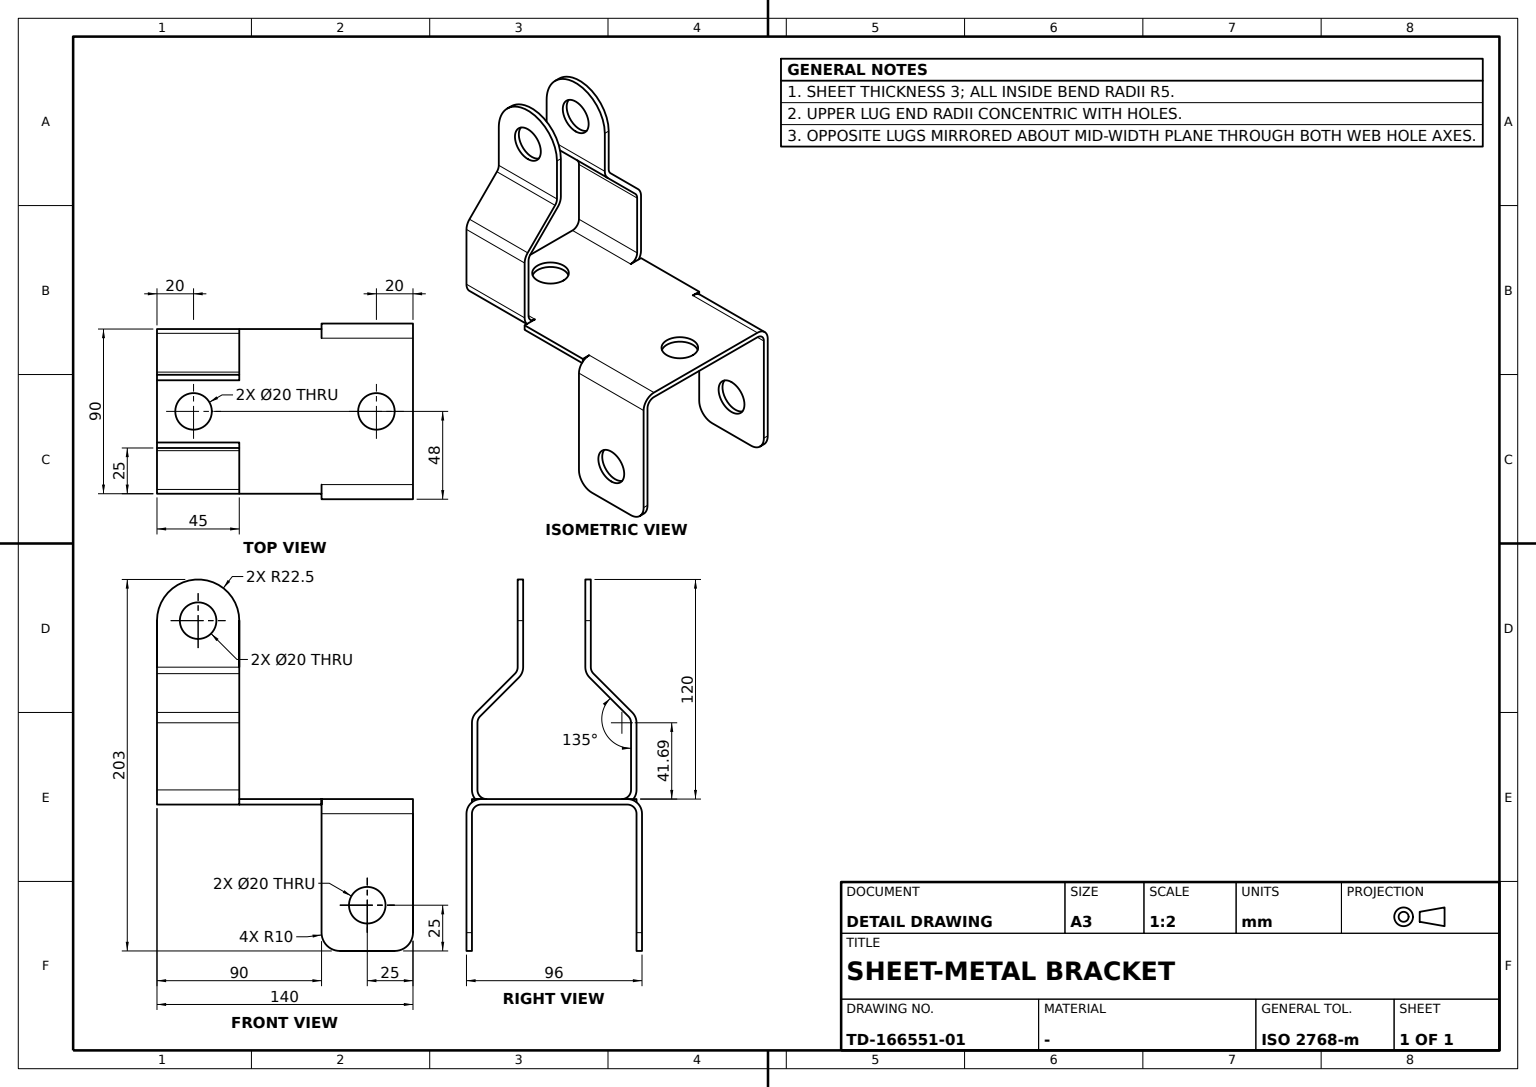
solid
v1 (60,0,1.5)
e1 v1 v1 CIRCLE(AX(P(50,0,1.5),D(0,0,1),D(1,0,0)),10)
v2 (60,0,-1.5)
e2 v2 v2 CIRCLE(AX(P(50,0,-1.5),D(0,0,1),D(1,0,0)),10)
face CYL(AX(P(50,0,-1.5),D(0,0,1),D(1,0,0)),10) rev [e1] [-e2]
v3 (45,48,-46.5)
e3 v3 v3 CIRCLE(AX(P(45,48,-56.5),D(0,1,0),D(0,0,1)),10) rev
v4 (45,45,-46.5)
e4 v4 v4 CIRCLE(AX(P(45,45,-56.5),D(0,1,0),D(0,0,1)),10)
face CYL(AX(P(45,48,-56.5),D(0,1,0),D(1,0,0)),10) rev [-e3] [-e4]
v5 (-25,-45,43.186292)
v6 (-70,-45,43.186292)
e5 v5 v6 LINE
v7 (-70,-45,6.5)
e6 v7 v6 LINE
v8 (-25,-45,6.5)
e7 v8 v7 LINE
e8 v8 v5 LINE
face PLANE(AX(P(-70,-45,1.5),D(0,-1,0),D(0,0,1))) [e5 -e6 -e7 e8]
v9 (30.000004,-45,-81.5)
v10 (60,-45,-81.5)
e9 v9 v10 LINE
v11 (60,-48,-81.5)
e10 v10 v11 LINE
v12 (30,-48,-81.5)
e11 v11 v12 LINE
e12 v9 v12 LINE
face PLANE(AX(P(45,48,-81.5),D(0,0,1),D(1,0,0))) rev [e9 e10 e11 -e12]
v13 (-70,-20,73.571068)
v14 (-70,-20,99)
e13 v13 v14 LINE
v15 (-25,-20,73.571068)
e14 v15 v13 LINE
v16 (-25,-20,99)
e15 v15 v16 LINE
e16 v16 v14 CIRCLE(AX(P(-47.5,-20,99),D(0,-1,0),D(0,0,-1)),22.5)
v17 (-47.5,-20,89)
e17 v17 v17 CIRCLE(AX(P(-47.5,-20,99),D(0,-1,0),D(0,0,-1)),10)
face PLANE(AX(P(-70,-20,71.5),D(0,-1,0),D(0,0,1))) [-e13 -e14 e15 e16] [-e17]
v18 (30,48,-81.5)
v19 (60,48,-81.5)
e18 v18 v19 LINE
v20 (20,48,-71.5)
e19 v18 v20 CIRCLE(AX(P(30,48,-71.5),D(0,1,0),D(0,0,1)),10)
v21 (20,48,-6.5)
e20 v20 v21 LINE
v22 (70,48,-6.5)
e21 v21 v22 LINE
v23 (70,48,-71.5)
e22 v23 v22 LINE
e23 v23 v19 CIRCLE(AX(P(60,48,-71.5),D(0,1,0),D(0,0,1)),10)
face PLANE(AX(P(0,48,-1.5),D(0,1,0),D(1,0,0))) [e3] [-e18 e19 e20 e21 -e22 e23]
v24 (20,-40,-1.5)
v25 (20,-45,-6.5)
e24 v24 v25 CIRCLE(AX(P(20,-40,-6.5),D(1,0,0),D(0,1,0)),5)
v26 (70,-40,-1.5)
e25 v26 v24 LINE
v27 (70,-45,-6.5)
e26 v27 v26 CIRCLE(AX(P(70,-40,-6.5),D(-1,0,0),D(0,0,1)),5)
e27 v27 v25 LINE
face CYL(AX(P(0,-40,-6.5),D(-1,0,0),D(0,0,1)),5) rev [-e24 -e25 -e26 e27]
v28 (-25,-42.656854,48.843146)
e28 v28 v5 CIRCLE(AX(P(-25,-37,43.186292),D(-1,0,0),D(0,0,1)),8) rev
v29 (-70,-42.656854,48.843146)
e29 v28 v29 LINE
e30 v6 v29 CIRCLE(AX(P(-70,-37,43.186292),D(-1,0,0),D(0,0,1)),8)
face CYL(AX(P(-47.5,-37,43.186292),D(1,0,0),D(0,-1,0)),8) [-e5 -e28 e29 -e30]
v30 (-70,-17,99)
e31 v14 v30 LINE
v31 (-25,-17,99)
e32 v16 v31 LINE
e33 v31 v30 CIRCLE(AX(P(-47.5,-17,99),D(0,-1,0),D(0,0,-1)),22.5)
face CYL(AX(P(-47.5,-20,99),D(0,-1,0),D(0,0,1)),22.5) [-e31 -e16 e32 e33]
v32 (-25,-37,-1.5)
v33 (-25,-37,1.5)
e34 v32 v33 LINE
v34 (-25,-45,-1.5)
e35 v34 v32 LINE
v35 (-25,-45,1.5)
e36 v34 v35 LINE
e37 v35 v33 LINE
face PLANE(AX(P(-25,31,58.37868),D(-1,0,0),D(0,1,0))) [-e34 -e35 e36 e37]
v36 (-25,-21.464466,70.035534)
v37 (-70,-21.464466,70.035534)
e38 v36 v37 LINE
e39 v29 v37 LINE
e40 v28 v36 LINE
face PLANE(AX(P(-70,-45,46.5),D(0,-0.707106781,0.707106781),D(0,0.707106781,0.707106781))) [e38 -e39 -e29 e40]
v38 (-25,37,-1.5)
v39 (-25,45,6.5)
e41 v38 v39 CIRCLE(AX(P(-25,37,6.5),D(-1,0,0),D(0,0,1)),8) rev
v40 (-70,37,-1.5)
e42 v38 v40 LINE
v41 (-70,45,6.5)
e43 v40 v41 CIRCLE(AX(P(-70,37,6.5),D(-1,0,0),D(0,0,1)),8) rev
e44 v39 v41 LINE
face CYL(AX(P(0,37,6.5),D(-1,0,0),D(0,0,-1)),8) [-e41 e42 e43 -e44]
v42 (-25,40.535534,46.721825)
v43 (-70,40.535534,46.721825)
e45 v42 v43 LINE
v44 (-70,42,43.186292)
e46 v44 v43 CIRCLE(AX(P(-70,37,43.186292),D(-1,0,0),D(0,0,1)),5) rev
v45 (-25,42,43.186292)
e47 v45 v44 LINE
e48 v42 v45 CIRCLE(AX(P(-25,37,43.186292),D(-1,0,0),D(0,0,1)),5)
face CYL(AX(P(-47.5,37,43.186292),D(-1,0,0),D(0,1,0)),5) rev [e45 -e46 -e47 -e48]
v46 (30,45,-81.5)
e49 v46 v18 LINE
v47 (20,45,-71.499996)
e50 v46 v47 CIRCLE(AX(P(30,45,-71.5),D(0,1,0),D(0,0,1)),10)
e51 v47 v20 LINE
face CYL(AX(P(30,45,-71.5),D(0,1,0),D(1,0,0)),10) [-e49 e50 e51 -e19]
v48 (-25,-42,43.186292)
v49 (-70,-42,43.186292)
e52 v48 v49 LINE
v50 (-70,-40.535534,46.721825)
e53 v49 v50 CIRCLE(AX(P(-70,-37,43.186292),D(-1,0,0),D(0,0,1)),5)
v51 (-25,-40.535534,46.721825)
e54 v51 v50 LINE
e55 v51 v48 CIRCLE(AX(P(-25,-37,43.186292),D(-1,0,0),D(0,0,1)),5) rev
face CYL(AX(P(-47.5,-37,43.186292),D(1,0,0),D(0,-1,0)),5) rev [e52 e53 -e54 e55]
v52 (-25,42.656854,48.843146)
v53 (-25,21.464466,70.035534)
e56 v52 v53 LINE
v54 (-70,42.656854,48.843146)
e57 v52 v54 LINE
v55 (-70,21.464466,70.035534)
e58 v54 v55 LINE
e59 v53 v55 LINE
face PLANE(AX(P(-70,45,46.5),D(0,-0.707106781,-0.707106781),D(0,-0.707106781,0.707106781))) rev [-e56 e57 e58 -e59]
v56 (59.999996,45,-81.5)
e60 v56 v19 LINE
e61 v56 v46 LINE
face PLANE(AX(P(45,48,-81.5),D(0,0,1),D(1,0,0))) rev [e49 e18 -e60 e61]
v57 (-25,20,73.571068)
e62 v53 v57 CIRCLE(AX(P(-25,25,73.571068),D(-1,0,0),D(0,0,1)),5)
v58 (-25,20,99)
e63 v57 v58 LINE
v59 (-25,17,99)
e64 v58 v59 LINE
v60 (-25,17,73.571068)
e65 v60 v59 LINE
v61 (-25,19.343146,67.914214)
e66 v61 v60 CIRCLE(AX(P(-25,25,73.571068),D(-1,0,0),D(0,0,1)),8)
e67 v42 v61 LINE
v62 (-25,42,6.5)
e68 v62 v45 LINE
v63 (-25,37,1.5)
e69 v63 v62 CIRCLE(AX(P(-25,37,6.5),D(-1,0,0),D(0,0,1)),5) rev
e70 v38 v63 LINE
v64 (-25,45,43.186292)
e71 v39 v64 LINE
e72 v52 v64 CIRCLE(AX(P(-25,37,43.186292),D(-1,0,0),D(0,0,1)),8)
face PLANE(AX(P(-25,31,58.37868),D(-1,0,0),D(0,1,0))) rev [e62 e63 e64 -e65 -e66 -e67 e48 -e68 -e69 -e70 e41 e71 -e72 e56]
v65 (20,-45,-1.5)
v66 (20,-45,1.5)
e73 v65 v66 LINE
e74 v35 v66 LINE
e75 v34 v65 LINE
face PLANE(AX(P(-70,-45,1.5),D(0,-1,0),D(0,0,1))) [e73 -e74 -e36 e75]
e76 v36 v15 CIRCLE(AX(P(-25,-25,73.571068),D(-1,0,0),D(0,0,1)),5) rev
e77 v32 v8 CIRCLE(AX(P(-25,-37,6.5),D(-1,0,0),D(0,0,1)),8)
v67 (-25,-42,6.5)
e78 v33 v67 CIRCLE(AX(P(-25,-37,6.5),D(-1,0,0),D(0,0,1)),5)
e79 v67 v48 LINE
v68 (-25,-19.343146,67.914214)
e80 v51 v68 LINE
v69 (-25,-17,73.571068)
e81 v68 v69 CIRCLE(AX(P(-25,-25,73.571068),D(-1,0,0),D(0,0,1)),8) rev
e82 v69 v31 LINE
face PLANE(AX(P(-25,31,58.37868),D(-1,0,0),D(0,1,0))) rev [-e32 -e15 -e76 -e40 e28 -e8 -e77 e34 e78 e79 -e55 e80 e81 e82]
e83 v13 v37 CIRCLE(AX(P(-70,-25,73.571068),D(-1,0,0),D(0,0,1)),5)
face CYL(AX(P(-47.5,-25,73.571068),D(1,0,0),D(0,0.707106781,-0.707106781)),5) rev [e76 e14 e83 -e38]
v70 (-25,45,-1.5)
v71 (-25,45,1.5)
e84 v70 v71 LINE
e85 v38 v70 LINE
e86 v63 v71 LINE
face PLANE(AX(P(-25,31,58.37868),D(-1,0,0),D(0,1,0))) [-e84 -e85 e70 e86]
e87 v65 v24 LINE
v72 (20,-40,1.5)
e88 v24 v72 LINE
e89 v66 v72 LINE
face PLANE(AX(P(20,42.5,1.5),D(1,0,0),D(0,1,0))) [-e73 e87 e88 -e89]
v73 (-47.5,-17,89)
e90 v73 v73 CIRCLE(AX(P(-47.5,-17,99),D(0,-1,0),D(0,0,-1)),10) rev
v74 (-70,-17,73.571068)
e91 v69 v74 LINE
e92 v74 v30 LINE
face PLANE(AX(P(-70,-17,71.5),D(0,-1,0),D(0,0,1))) rev [-e90] [-e82 e91 e92 -e33]
face CYL(AX(P(-47.5,-20,99),D(0,-1,0),D(0,0,1)),10) rev [e90] [e17]
v75 (-70,-42,6.5)
e93 v67 v75 LINE
e94 v75 v49 LINE
face PLANE(AX(P(-70,-42,1.5),D(0,-1,0),D(0,0,1))) rev [e93 e94 -e52 -e79]
v76 (70,-48,-6.5)
v77 (70,-40,1.5)
e95 v76 v77 CIRCLE(AX(P(70,-40,-6.5),D(-1,0,0),D(0,0,1)),8)
e96 v77 v72 LINE
v78 (20,-48,-6.5)
e97 v72 v78 CIRCLE(AX(P(20,-40,-6.5),D(1,0,0),D(0,1,0)),8)
e98 v76 v78 LINE
face CYL(AX(P(0,-40,-6.5),D(-1,0,0),D(0,0,1)),8) [e95 e96 e97 -e98]
v79 (20,45,-6.5)
e99 v79 v47 LINE
v80 (70,45,-71.5)
e100 v80 v56 CIRCLE(AX(P(60,45,-71.5),D(0,1,0),D(0,0,1)),10)
v81 (70,45,-6.5)
e101 v81 v80 LINE
e102 v79 v81 LINE
face PLANE(AX(P(70,45,-1.5),D(0,1,0),D(-1,0,0))) rev [e4] [e99 -e50 -e61 -e100 -e101 -e102]
v82 (-40,0,1.5)
e103 v82 v82 CIRCLE(AX(P(-50,0,1.5),D(0,0,1),D(1,0,0)),10)
v83 (-40,0,-1.5)
e104 v83 v83 CIRCLE(AX(P(-50,0,-1.5),D(0,0,1),D(1,0,0)),10)
face CYL(AX(P(-50,0,-1.5),D(0,0,1),D(1,0,0)),10) rev [e103] [-e104]
v84 (20,45,1.5)
e105 v84 v71 LINE
v85 (20,45,-1.5)
e106 v85 v84 LINE
e107 v85 v70 LINE
face PLANE(AX(P(70,45,-1.5),D(0,1,0),D(-1,0,0))) [e84 -e105 -e106 e107]
v86 (-70,42,6.5)
e108 v62 v86 LINE
v87 (-70,37,1.5)
e109 v87 v86 CIRCLE(AX(P(-70,37,6.5),D(-1,0,0),D(0,0,1)),5) rev
e110 v63 v87 LINE
face CYL(AX(P(0,37,6.5),D(-1,0,0),D(0,0,-1)),5) rev [e108 -e109 -e110 e69]
v88 (-70,-19.343146,67.914214)
e111 v74 v88 CIRCLE(AX(P(-70,-25,73.571068),D(-1,0,0),D(0,0,1)),8)
e112 v50 v88 LINE
v89 (-70,-37,1.5)
e113 v75 v89 CIRCLE(AX(P(-70,-37,6.5),D(-1,0,0),D(0,0,1)),5) rev
e114 v87 v89 LINE
e115 v86 v44 LINE
v90 (-70,19.343146,67.914214)
e116 v43 v90 LINE
v91 (-70,17,73.571068)
e117 v91 v90 CIRCLE(AX(P(-70,25,73.571068),D(-1,0,0),D(0,0,1)),8) rev
v92 (-70,17,99)
e118 v91 v92 LINE
v93 (-70,20,99)
e119 v93 v92 LINE
v94 (-70,20,73.571068)
e120 v94 v93 LINE
e121 v94 v55 CIRCLE(AX(P(-70,25,73.571068),D(-1,0,0),D(0,0,1)),5) rev
v95 (-70,45,43.186292)
e122 v95 v54 CIRCLE(AX(P(-70,37,43.186292),D(-1,0,0),D(0,0,1)),8) rev
e123 v41 v95 LINE
v96 (-70,-37,-1.5)
e124 v40 v96 LINE
e125 v7 v96 CIRCLE(AX(P(-70,-37,6.5),D(-1,0,0),D(0,0,1)),8) rev
face PLANE(AX(P(-70,18.5,97.535534),D(-1,0,0),D(0,1,0))) [e13 e31 -e92 e111 -e112 -e53 -e94 e113 -e114 e109 e115 e46 e116 -e117 e118 -e119 -e120 e121 -e58 -e122 -e123 -e43 e124 -e125 e6 e30 e39 -e83]
v97 (20,40,1.5)
v98 (70,40,1.5)
e126 v97 v98 LINE
e127 v22 v98 CIRCLE(AX(P(70,40,-6.5),D(-1,0,0),D(0,0,1)),8) rev
e128 v97 v21 CIRCLE(AX(P(20,40,-6.5),D(1,0,0),D(0,1,0)),8) rev
face CYL(AX(P(0,40,-6.5),D(1,0,0),D(0,0,1)),8) [e126 -e127 -e21 -e128]
v99 (45,-48,-66.5)
e129 v99 v99 CIRCLE(AX(P(45,-48,-56.5),D(0,-1,0),D(0,0,-1)),10)
v100 (45,-45,-66.5)
e130 v100 v100 CIRCLE(AX(P(45,-45,-56.5),D(0,-1,0),D(0,0,-1)),10)
face CYL(AX(P(45,48,-56.5),D(0,1,0),D(1,0,0)),10) rev [e129] [-e130]
v101 (-47.5,17,89)
e131 v101 v101 CIRCLE(AX(P(-47.5,17,99),D(0,-1,0),D(0,0,-1)),10)
v102 (-47.5,20,89)
e132 v102 v102 CIRCLE(AX(P(-47.5,20,99),D(0,-1,0),D(0,0,-1)),10)
face CYL(AX(P(-47.5,-20,99),D(0,-1,0),D(0,0,1)),10) rev [e131] [-e132]
v103 (20,40,-1.5)
e133 v103 v79 CIRCLE(AX(P(20,40,-6.5),D(1,0,0),D(0,1,0)),5) rev
e134 v103 v97 LINE
face PLANE(AX(P(20,42.5,1.5),D(1,0,0),D(0,1,0))) rev [-e20 -e51 -e99 -e133 e134 e128]
e135 v68 v88 LINE
face CYL(AX(P(-47.5,-25,73.571068),D(1,0,0),D(0,0.707106781,-0.707106781)),8) [-e81 e135 -e111 -e91]
v104 (20,-45,-71.5)
e136 v104 v9 CIRCLE(AX(P(30,-45,-71.5),D(0,-1,0),D(0,0,-1)),10)
v105 (20,-48,-71.499996)
e137 v105 v12 CIRCLE(AX(P(30,-48,-71.5),D(0,-1,0),D(0,0,-1)),10)
e138 v104 v105 LINE
face CYL(AX(P(30,45,-71.5),D(0,1,0),D(1,0,0)),10) [e136 e12 -e137 -e138]
e139 v57 v94 LINE
e140 v58 v93 CIRCLE(AX(P(-47.5,20,99),D(0,-1,0),D(0,0,-1)),22.5)
face PLANE(AX(P(-70,20,71.5),D(0,-1,0),D(0,0,1))) rev [e139 e120 -e140 -e63] [e132]
e141 v77 v98 LINE
v106 (70,-48,-71.5)
e142 v106 v76 LINE
v107 (70,-45,-71.499996)
e143 v107 v106 LINE
e144 v27 v107 LINE
v108 (70,40,-1.5)
e145 v26 v108 LINE
e146 v81 v108 CIRCLE(AX(P(70,40,-6.5),D(-1,0,0),D(0,0,1)),5) rev
e147 v80 v23 LINE
face PLANE(AX(P(70,48,-44),D(-1,0,0),D(0,1,0))) rev [e22 e127 -e141 -e95 -e142 -e143 -e144 e26 e145 -e146 e101 e147]
e148 v60 v91 LINE
e149 v61 v90 LINE
face CYL(AX(P(-47.5,25,73.571068),D(-1,0,0),D(0,-0.707106781,-0.707106781)),8) [e66 e148 e117 -e149]
e150 v32 v96 LINE
face CYL(AX(P(0,-37,6.5),D(-1,0,0),D(0,-1,0)),8) [-e150 e77 e7 e125]
e151 v105 v78 LINE
e152 v11 v106 CIRCLE(AX(P(60,-48,-71.5),D(0,-1,0),D(0,0,-1)),10)
face PLANE(AX(P(0,-48,-1.5),D(0,-1,0),D(-1,0,0))) [-e129] [e142 e98 -e151 e137 -e11 e152]
face CYL(AX(P(-47.5,25,73.571068),D(-1,0,0),D(0,-0.707106781,-0.707106781)),5) rev [-e62 e59 -e121 -e139]
face PLANE(AX(P(-70,42.87868,44.37868),D(0,-0.707106781,-0.707106781),D(0,-0.707106781,0.707106781))) [e149 -e116 -e45 e67]
e153 v64 v95 LINE
face PLANE(AX(P(70,45,-1.5),D(0,1,0),D(-1,0,0))) [e123 -e153 -e71 e44]
face CYL(AX(P(60,45,-71.5),D(0,1,0),D(1,0,0)),10) [e60 -e23 -e147 e100]
face PLANE(AX(P(-70,-42.87868,44.37868),D(0,-0.707106781,0.707106781),D(0,0.707106781,0.707106781))) rev [-e80 e54 e112 -e135]
e154 v84 v97 LINE
e155 v85 v103 LINE
face PLANE(AX(P(20,42.5,1.5),D(1,0,0),D(0,1,0))) [e154 -e134 -e155 e106]
e156 v103 v108 LINE
face CYL(AX(P(0,40,-6.5),D(1,0,0),D(0,0,1)),5) rev [-e156 e133 e102 e146]
face PLANE(AX(P(0,0,-1.5),D(0,0,1),D(1,0,0))) rev [e2] [-e42 e85 -e107 e155 e156 -e145 e25 -e87 -e75 e35 e150 -e124] [e104]
face CYL(AX(P(-47.5,37,43.186292),D(-1,0,0),D(0,1,0)),8) [e122 -e57 e72 e153]
e157 v25 v104 LINE
face PLANE(AX(P(20,42.5,1.5),D(1,0,0),D(0,1,0))) rev [e24 e157 e138 e151 -e97 -e88]
e158 v59 v92 CIRCLE(AX(P(-47.5,17,99),D(0,-1,0),D(0,0,-1)),22.5)
face PLANE(AX(P(-70,17,71.5),D(0,-1,0),D(0,0,1))) [-e131] [e158 -e118 -e148 e65]
e159 v10 v107 CIRCLE(AX(P(60,-45,-71.5),D(0,-1,0),D(0,0,-1)),10)
face PLANE(AX(P(-70,-45,1.5),D(0,-1,0),D(0,0,1))) rev [e130] [e144 -e159 -e9 -e136 -e157 -e27]
e160 v33 v89 LINE
face CYL(AX(P(0,-37,6.5),D(-1,0,0),D(0,-1,0)),5) rev [-e93 -e78 e160 -e113]
face PLANE(AX(P(-70,42,1.5),D(0,-1,0),D(0,0,1))) [-e108 e68 e47 -e115]
face CYL(AX(P(-47.5,-20,99),D(0,-1,0),D(0,0,1)),22.5) [-e158 -e64 e140 e119]
face PLANE(AX(P(0,0,1.5),D(0,0,1),D(1,0,0))) [-e103] [-e1] [e141 -e126 -e154 e105 -e86 e110 e114 -e160 -e37 e74 e89 -e96]
face CYL(AX(P(60,45,-71.5),D(0,1,0),D(1,0,0)),10) [-e10 e159 e143 -e152]
